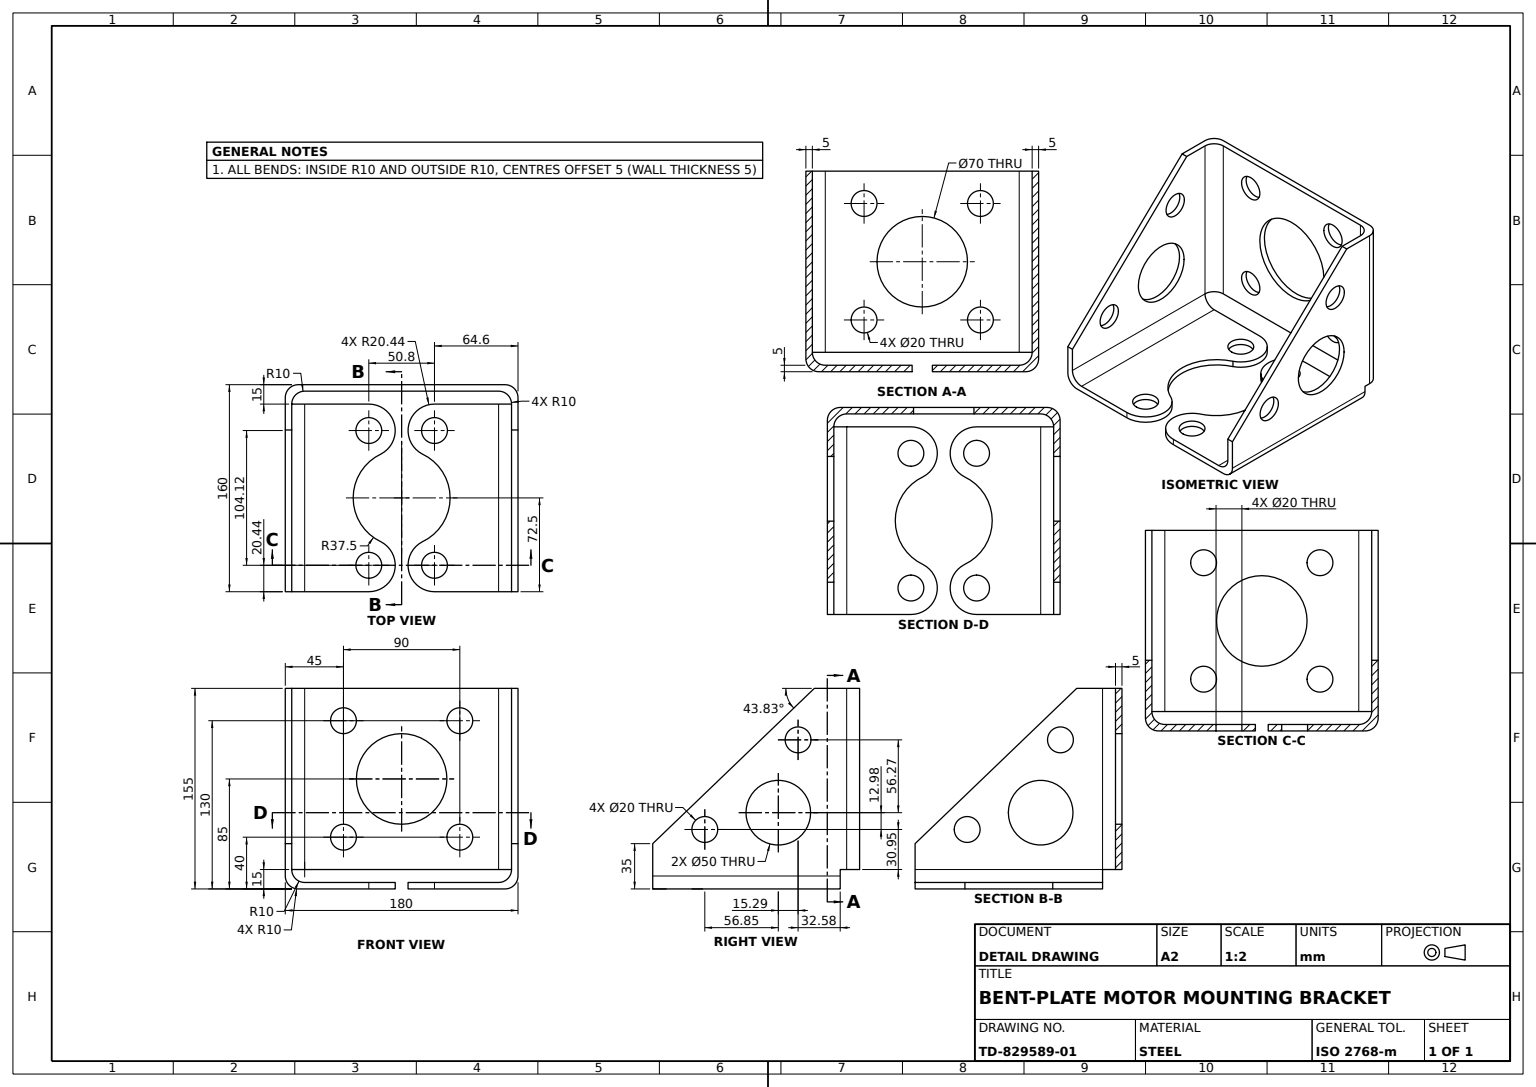
solid
v1 (75,-80,15)
v2 (85,-70,15)
e1 v1 v2 CIRCLE(AX(P(75,-70,15),D(0,0,1),D(1,0,0)),10)
v3 (75,-80,160)
e2 v3 v1 LINE
v4 (85,-70,160)
e3 v4 v3 CIRCLE(AX(P(75,-70,160),D(0,0,-1),D(-1,0,0)),10)
e4 v2 v4 LINE
face CYL(AX(P(75,-70,0),D(0,0,1),D(1,0,0)),10) rev [-e1 -e2 -e3 -e4]
v5 (-85,-26.069366,37.873409)
v6 (-90,-26.069366,37.873409)
e5 v5 v6 LINE
v7 (-85,-26.069366,87.873409)
e6 v7 v5 CIRCLE(AX(P(-85,-26.069366,62.873409),D(-1,0,0),D(0,0,1)),25)
v8 (-90,-26.069366,87.873409)
e7 v7 v8 LINE
e8 v8 v6 CIRCLE(AX(P(-90,-26.069366,62.873409),D(-1,0,0),D(0,0,1)),25)
face CYL(AX(P(-85,-26.069366,62.873409),D(-1,0,0),D(0,0,1)),25) rev [-e5 -e6 e7 e8]
v9 (-25.4,-80,129.56)
v10 (-25.4,-80,149.56)
e9 v9 v10 CIRCLE(AX(P(-25.4,-80,139.56),D(0,-1,0),D(0,0,-1)),10)
e10 v10 v9 CIRCLE(AX(P(-25.4,-80,139.56),D(0,-1,0),D(0,0,-1)),10)
v11 (-75,-80,15)
v12 (-75,-80,160)
e11 v11 v12 LINE
v13 (-25.4,-80,160)
e12 v12 v13 LINE
v14 (-15.8913,-80,121.466404)
e13 v14 v13 CIRCLE(AX(P(-25.4,-80,139.56),D(0,-1,0),D(0,0,-1)),20.44)
v15 (-15.8913,-80,53.533596)
e14 v14 v15 CIRCLE(AX(P(0,-80,87.5),D(0,-1,0),D(0,0,-1)),37.5)
v16 (-25.4,-80,15)
e15 v16 v15 CIRCLE(AX(P(-25.4,-80,35.44),D(0,-1,0),D(0,0,-1)),20.44)
e16 v11 v16 LINE
v17 (-25.4,-80,45.44)
v18 (-25.4,-80,25.44)
e17 v17 v18 CIRCLE(AX(P(-25.4,-80,35.44),D(0,-1,0),D(0,0,-1)),10)
e18 v18 v17 CIRCLE(AX(P(-25.4,-80,35.44),D(0,-1,0),D(0,0,-1)),10)
face PLANE(AX(P(0,-80,0),D(0,-1,0),D(0,0,-1))) rev [e9 e10] [e11 e12 -e13 e14 -e15 -e16] [e17 e18]
v19 (-85,-70,15)
e19 v19 v11 CIRCLE(AX(P(-75,-70,15),D(0,0,1),D(1,0,0)),10)
v20 (-85,-70,160)
e20 v20 v19 LINE
e21 v12 v20 CIRCLE(AX(P(-75,-70,160),D(0,0,-1),D(1,0,0)),10)
face CYL(AX(P(-75,-70,0),D(0,0,-1),D(-1,0,0)),10) rev [-e11 -e19 -e20 -e21]
v21 (85,-39.054338,129.718729)
v22 (90,-39.054338,129.718729)
e22 v21 v22 LINE
v23 (85,-39.054338,109.718729)
e23 v21 v23 CIRCLE(AX(P(85,-39.054338,119.718729),D(-1,0,0),D(0,0,1)),10)
v24 (90,-39.054338,109.718729)
e24 v23 v24 LINE
e25 v22 v24 CIRCLE(AX(P(90,-39.054338,119.718729),D(-1,0,0),D(0,0,1)),10)
face CYL(AX(P(85,-39.054338,119.718729),D(1,0,0),D(0,0,-1)),10) rev [-e22 e23 e24 -e25]
v25 (-85,-39.054338,109.718729)
v26 (-85,-39.054338,129.718729)
e26 v25 v26 CIRCLE(AX(P(-85,-39.054338,119.718729),D(-1,0,0),D(0,0,1)),10)
e27 v26 v25 CIRCLE(AX(P(-85,-39.054338,119.718729),D(-1,0,0),D(0,0,1)),10)
v27 (-85,70,15)
v28 (-85,70,35)
e28 v27 v28 LINE
v29 (-85,-50,160)
e29 v29 v28 LINE
e30 v20 v29 LINE
e31 v19 v27 LINE
e32 v5 v7 CIRCLE(AX(P(-85,-26.069366,62.873409),D(-1,0,0),D(0,0,1)),25)
v30 (-85,30.198845,57.579997)
v31 (-85,30.198845,37.579997)
e33 v30 v31 CIRCLE(AX(P(-85,30.198845,47.579997),D(-1,0,0),D(0,0,1)),10)
e34 v31 v30 CIRCLE(AX(P(-85,30.198845,47.579997),D(-1,0,0),D(0,0,1)),10)
face PLANE(AX(P(-85,0,0),D(-1,0,0),D(0,0,1))) rev [e26 e27] [e28 -e29 -e30 e20 e31] [e32 e6] [e33 e34]
v32 (25.4,-80,15)
e35 v32 v1 LINE
v33 (15.8913,-80,53.533596)
e36 v33 v32 CIRCLE(AX(P(25.4,-80,35.44),D(0,-1,0),D(0,0,-1)),20.44)
v34 (15.8913,-80,121.466404)
e37 v33 v34 CIRCLE(AX(P(0,-80,87.5),D(0,-1,0),D(0,0,-1)),37.5)
v35 (25.4,-80,160)
e38 v35 v34 CIRCLE(AX(P(25.4,-80,139.56),D(0,-1,0),D(0,0,-1)),20.44)
e39 v35 v3 LINE
v36 (25.4,-80,45.44)
v37 (25.4,-80,25.44)
e40 v36 v37 CIRCLE(AX(P(25.4,-80,35.44),D(0,-1,0),D(0,0,-1)),10)
e41 v37 v36 CIRCLE(AX(P(25.4,-80,35.44),D(0,-1,0),D(0,0,-1)),10)
v38 (25.4,-80,149.56)
v39 (25.4,-80,129.56)
e42 v38 v39 CIRCLE(AX(P(25.4,-80,139.56),D(0,-1,0),D(0,0,-1)),10)
e43 v39 v38 CIRCLE(AX(P(25.4,-80,139.56),D(0,-1,0),D(0,0,-1)),10)
face PLANE(AX(P(0,-80,0),D(0,-1,0),D(0,0,-1))) rev [e2 -e35 -e36 e37 -e38 e39] [e40 e41] [e42 e43]
v40 (90,-70,15)
e44 v2 v40 LINE
v41 (90,-75,15)
e45 v41 v40 LINE
v42 (80,-85,15)
e46 v41 v42 CIRCLE(AX(P(80,-75,15),D(0,0,-1),D(1,0,0)),10)
v43 (25.4,-85,15)
e47 v43 v42 LINE
e48 v32 v43 LINE
face PLANE(AX(P(85,-85,15),D(0,0,1),D(1,0,0))) rev [e35 e1 e44 -e45 e46 -e47 -e48]
v44 (-15.8913,-85,121.466404)
e49 v14 v44 LINE
v45 (-25.4,-85,160)
e50 v13 v45 LINE
e51 v44 v45 CIRCLE(AX(P(-25.4,-85,139.56),D(0,-1,0),D(0,0,-1)),20.44)
face CYL(AX(P(-25.4,-80,139.56),D(0,-1,0),D(0,0,-1)),20.44) [-e49 e13 e50 -e51]
v46 (90,-26.069366,37.873409)
v47 (90,-26.069366,87.873409)
e52 v46 v47 CIRCLE(AX(P(90,-26.069366,62.873409),D(-1,0,0),D(0,0,1)),25)
v48 (85,-26.069366,37.873409)
e53 v48 v46 LINE
v49 (85,-26.069366,87.873409)
e54 v48 v49 CIRCLE(AX(P(85,-26.069366,62.873409),D(-1,0,0),D(0,0,1)),25)
e55 v49 v47 LINE
face CYL(AX(P(85,-26.069366,62.873409),D(1,0,0),D(0,0,-1)),25) rev [-e52 -e53 e54 e55]
v50 (25.4,-85,45.44)
v51 (25.4,-85,25.44)
e56 v50 v51 CIRCLE(AX(P(25.4,-85,35.44),D(0,-1,0),D(0,0,-1)),10)
e57 v37 v51 LINE
e58 v36 v50 LINE
face CYL(AX(P(25.4,-80,35.44),D(0,-1,0),D(0,0,-1)),10) rev [e56 -e57 -e40 e58]
e59 v23 v21 CIRCLE(AX(P(85,-39.054338,119.718729),D(-1,0,0),D(0,0,1)),10)
e60 v24 v22 CIRCLE(AX(P(90,-39.054338,119.718729),D(-1,0,0),D(0,0,1)),10)
face CYL(AX(P(85,-39.054338,119.718729),D(1,0,0),D(0,0,-1)),10) rev [e59 e22 -e60 -e24]
v52 (-55,-45,5)
v53 (-35,-45,5)
e61 v52 v53 CIRCLE(AX(P(-45,-45,5),D(0,0,1),D(1,0,0)),10)
v54 (-35,-45,0)
e62 v53 v54 LINE
v55 (-55,-45,0)
e63 v55 v54 CIRCLE(AX(P(-45,-45,0),D(0,0,1),D(1,0,0)),10)
e64 v52 v55 LINE
face CYL(AX(P(-45,-45,5),D(0,0,-1),D(-1,0,0)),10) rev [e61 e62 -e63 -e64]
e65 v6 v8 CIRCLE(AX(P(-90,-26.069366,62.873409),D(-1,0,0),D(0,0,1)),25)
v56 (-90,70,35)
v57 (-90,70,10)
e66 v56 v57 LINE
v58 (-90,-70,10)
e67 v57 v58 LINE
v59 (-90,-70,15)
e68 v59 v58 LINE
v60 (-90,-75,15)
e69 v60 v59 LINE
v61 (-90,-75,160)
e70 v60 v61 LINE
v62 (-90,-50,160)
e71 v61 v62 LINE
e72 v62 v56 LINE
v63 (-90,30.198845,37.579997)
v64 (-90,30.198845,57.579997)
e73 v63 v64 CIRCLE(AX(P(-90,30.198845,47.579997),D(-1,0,0),D(0,0,1)),10)
e74 v64 v63 CIRCLE(AX(P(-90,30.198845,47.579997),D(-1,0,0),D(0,0,1)),10)
v65 (-90,-39.054338,109.718729)
v66 (-90,-39.054338,129.718729)
e75 v65 v66 CIRCLE(AX(P(-90,-39.054338,119.718729),D(-1,0,0),D(0,0,1)),10)
e76 v66 v65 CIRCLE(AX(P(-90,-39.054338,119.718729),D(-1,0,0),D(0,0,1)),10)
face PLANE(AX(P(-90,-70,5),D(1,0,0),D(0,0,-1))) rev [-e8 -e65] [e66 e67 -e68 -e69 e70 e71 e72] [-e73 -e74] [-e75 -e76]
v67 (75,-70,5)
e77 v2 v67 CIRCLE(AX(P(75,-70,15),D(0,1,0),D(0,0,1)),10)
v68 (-75,-70,5)
e78 v68 v67 LINE
e79 v68 v19 CIRCLE(AX(P(-75,-70,15),D(0,1,0),D(0,0,1)),10)
e80 v59 v19 LINE
v69 (-80,-70,0)
e81 v58 v69 CIRCLE(AX(P(-80,-70,10),D(0,-1,0),D(0,0,1)),10)
v70 (80,-70,0)
e82 v69 v70 LINE
v71 (90,-70,10)
e83 v70 v71 CIRCLE(AX(P(80,-70,10),D(0,-1,0),D(0,0,1)),10)
e84 v40 v71 LINE
face PLANE(AX(P(-90,-70,5),D(0,1,0),D(0,0,1))) rev [e77 -e78 e79 -e80 e68 e81 e82 e83 -e84 -e44]
v72 (25.4,-85,149.56)
e85 v38 v72 LINE
v73 (25.4,-85,129.56)
e86 v39 v73 LINE
e87 v73 v72 CIRCLE(AX(P(25.4,-85,139.56),D(0,-1,0),D(0,0,-1)),10)
face CYL(AX(P(25.4,-80,139.56),D(0,-1,0),D(0,0,-1)),10) rev [-e85 -e43 e86 e87]
v74 (85,30.198845,37.579997)
v75 (85,30.198845,57.579997)
e88 v74 v75 CIRCLE(AX(P(85,30.198845,47.579997),D(-1,0,0),D(0,0,1)),10)
e89 v75 v74 CIRCLE(AX(P(85,30.198845,47.579997),D(-1,0,0),D(0,0,1)),10)
v76 (85,-50,160)
e90 v4 v76 LINE
v77 (85,70,35)
e91 v76 v77 LINE
v78 (85,70,15)
e92 v78 v77 LINE
e93 v78 v2 LINE
e94 v49 v48 CIRCLE(AX(P(85,-26.069366,62.873409),D(-1,0,0),D(0,0,1)),25)
face PLANE(AX(P(85,0,0),D(-1,0,0),D(0,0,1))) [-e88 -e89] [e90 e91 -e92 e93 e4] [-e23 -e59] [-e94 -e54]
e95 v30 v64 LINE
e96 v31 v63 LINE
face CYL(AX(P(-85,30.198845,47.579997),D(-1,0,0),D(0,0,1)),10) rev [-e95 -e34 e96 e73]
v79 (-25.4,-85,149.56)
e97 v10 v79 LINE
v80 (-25.4,-85,129.56)
e98 v9 v80 LINE
e99 v80 v79 CIRCLE(AX(P(-25.4,-85,139.56),D(0,-1,0),D(0,0,-1)),10)
face CYL(AX(P(-25.4,-80,139.56),D(0,-1,0),D(0,0,-1)),10) rev [-e97 -e9 e98 e99]
e100 v53 v52 CIRCLE(AX(P(-45,-45,5),D(0,0,1),D(1,0,0)),10)
e101 v54 v55 CIRCLE(AX(P(-45,-45,0),D(0,0,1),D(1,0,0)),10)
face CYL(AX(P(-45,-45,5),D(0,0,-1),D(-1,0,0)),10) rev [-e62 e100 e64 -e101]
v81 (55,-45,0)
v82 (35,-45,0)
e102 v81 v82 CIRCLE(AX(P(45,-45,0),D(0,0,1),D(1,0,0)),10)
v83 (55,-45,5)
e103 v83 v81 LINE
v84 (35,-45,5)
e104 v83 v84 CIRCLE(AX(P(45,-45,5),D(0,0,1),D(1,0,0)),10)
e105 v84 v82 LINE
face CYL(AX(P(45,-45,5),D(0,0,-1),D(-1,0,0)),10) rev [-e102 -e103 e104 e105]
v85 (-80,-85,160)
e106 v61 v85 CIRCLE(AX(P(-80,-75,160),D(0,0,1),D(1,0,0)),10)
e107 v45 v85 LINE
e108 v29 v62 LINE
face PLANE(AX(P(-85,0,160),D(0,0,1),D(1,0,0))) [e106 -e107 -e50 -e12 e21 e30 e108 -e71]
v86 (-55,45,0)
v87 (-35,45,0)
e109 v86 v87 CIRCLE(AX(P(-45,45,0),D(0,0,1),D(1,0,0)),10)
e110 v87 v86 CIRCLE(AX(P(-45,45,0),D(0,0,1),D(1,0,0)),10)
v88 (80,70,0)
v89 (-80,70,0)
e111 v88 v89 LINE
e112 v88 v70 LINE
e113 v69 v89 LINE
e114 v82 v81 CIRCLE(AX(P(45,-45,0),D(0,0,1),D(1,0,0)),10)
v90 (35,0,0)
v91 (-35,0,0)
e115 v90 v91 CIRCLE(AX(P(0,0,0),D(0,0,1),D(1,0,0)),35)
e116 v91 v90 CIRCLE(AX(P(0,0,0),D(0,0,1),D(1,0,0)),35)
v92 (35,45,0)
v93 (55,45,0)
e117 v92 v93 CIRCLE(AX(P(45,45,0),D(0,0,1),D(1,0,0)),10)
e118 v93 v92 CIRCLE(AX(P(45,45,0),D(0,0,1),D(1,0,0)),10)
face PLANE(AX(P(0,0,0),D(0,0,-1),D(-1,0,0))) [e109 e110] [e101 e63] [-e111 e112 -e82 e113] [e114 e102] [e115 e116] [e117 e118]
v94 (-25.4,-85,45.44)
v95 (-25.4,-85,25.44)
e119 v94 v95 CIRCLE(AX(P(-25.4,-85,35.44),D(0,-1,0),D(0,0,-1)),10)
e120 v18 v95 LINE
e121 v17 v94 LINE
face CYL(AX(P(-25.4,-80,35.44),D(0,-1,0),D(0,0,-1)),10) rev [e119 -e120 -e17 e121]
e122 v72 v73 CIRCLE(AX(P(25.4,-85,139.56),D(0,-1,0),D(0,0,-1)),10)
face CYL(AX(P(25.4,-80,139.56),D(0,-1,0),D(0,0,-1)),10) rev [e122 -e86 -e42 e85]
v96 (90,-75,160)
e123 v96 v41 LINE
v97 (80,-85,160)
e124 v97 v96 CIRCLE(AX(P(80,-75,160),D(0,0,1),D(-1,0,0)),10)
e125 v42 v97 LINE
face CYL(AX(P(80,-75,0),D(0,0,-1),D(-1,0,0)),10) [-e123 -e124 -e125 -e46]
v98 (90,30.198845,57.579997)
e126 v75 v98 LINE
v99 (90,30.198845,37.579997)
e127 v99 v98 CIRCLE(AX(P(90,30.198845,47.579997),D(-1,0,0),D(0,0,1)),10)
e128 v74 v99 LINE
face CYL(AX(P(85,30.198845,47.579997),D(1,0,0),D(0,0,-1)),10) rev [e126 -e127 -e128 e88]
v100 (35,45,5)
e129 v100 v92 LINE
v101 (55,45,5)
e130 v100 v101 CIRCLE(AX(P(45,45,5),D(0,0,1),D(1,0,0)),10)
e131 v101 v93 LINE
face CYL(AX(P(45,45,5),D(0,0,-1),D(-1,0,0)),10) rev [-e129 e130 e131 -e117]
e132 v95 v94 CIRCLE(AX(P(-25.4,-85,35.44),D(0,-1,0),D(0,0,-1)),10)
face CYL(AX(P(-25.4,-80,35.44),D(0,-1,0),D(0,0,-1)),10) rev [e120 e132 -e121 -e18]
e133 v89 v57 CIRCLE(AX(P(-80,70,10),D(0,1,0),D(0,0,-1)),10)
face CYL(AX(P(-80,-70,10),D(0,1,0),D(0,0,1)),10) [-e81 -e67 -e133 -e113]
v102 (-15.8913,-85,53.533596)
e134 v44 v102 CIRCLE(AX(P(0,-85,87.5),D(0,-1,0),D(0,0,-1)),37.5)
v103 (-80,-85,15)
e135 v85 v103 LINE
v104 (-25.4,-85,15)
e136 v103 v104 LINE
e137 v104 v102 CIRCLE(AX(P(-25.4,-85,35.44),D(0,-1,0),D(0,0,-1)),20.44)
e138 v79 v80 CIRCLE(AX(P(-25.4,-85,139.56),D(0,-1,0),D(0,0,-1)),10)
face PLANE(AX(P(0,-85,0),D(0,-1,0),D(0,0,-1))) [-e132 -e119] [-e134 e51 e107 e135 e136 e137] [-e99 -e138]
e139 v26 v66 LINE
e140 v25 v65 LINE
face CYL(AX(P(-85,-39.054338,119.718729),D(-1,0,0),D(0,0,1)),10) rev [e75 -e139 -e26 e140]
e141 v101 v100 CIRCLE(AX(P(45,45,5),D(0,0,1),D(1,0,0)),10)
face CYL(AX(P(45,45,5),D(0,0,-1),D(-1,0,0)),10) rev [e141 e129 -e118 -e131]
v105 (-35,45,5)
v106 (-55,45,5)
e142 v105 v106 CIRCLE(AX(P(-45,45,5),D(0,0,1),D(1,0,0)),10)
e143 v106 v86 LINE
e144 v105 v87 LINE
face CYL(AX(P(-45,45,5),D(0,0,-1),D(-1,0,0)),10) rev [e142 e143 -e110 -e144]
e145 v84 v83 CIRCLE(AX(P(45,-45,5),D(0,0,1),D(1,0,0)),10)
face CYL(AX(P(45,-45,5),D(0,0,-1),D(-1,0,0)),10) rev [-e105 e145 e103 -e114]
e146 v103 v60 CIRCLE(AX(P(-80,-75,15),D(0,0,-1),D(1,0,0)),10)
face CYL(AX(P(-80,-75,0),D(0,0,1),D(1,0,0)),10) [-e70 -e146 -e135 -e106]
v107 (25.4,-85,160)
v108 (15.8913,-85,121.466404)
e147 v107 v108 CIRCLE(AX(P(25.4,-85,139.56),D(0,-1,0),D(0,0,-1)),20.44)
e148 v35 v107 LINE
e149 v34 v108 LINE
face CYL(AX(P(25.4,-80,139.56),D(0,-1,0),D(0,0,-1)),20.44) [-e147 -e148 e38 e149]
face CYL(AX(P(-25.4,-80,139.56),D(0,-1,0),D(0,0,-1)),10) rev [-e98 -e10 e97 e138]
v109 (90,70,35)
e150 v77 v109 LINE
v110 (90,-50,160)
e151 v76 v110 LINE
e152 v110 v109 LINE
face PLANE(AX(P(85,17.843464,89.329725),D(0,-0.721387321,-0.692531828),D(0,0.692531828,-0.721387321))) rev [-e150 -e91 e151 e152]
v111 (15.8913,-85,53.533596)
e153 v33 v111 LINE
e154 v111 v43 CIRCLE(AX(P(25.4,-85,35.44),D(0,-1,0),D(0,0,-1)),20.44)
face CYL(AX(P(25.4,-80,35.44),D(0,-1,0),D(0,0,-1)),20.44) [-e153 e36 e48 -e154]
v112 (-75,70,5)
e155 v27 v112 CIRCLE(AX(P(-75,70,15),D(0,-1,0),D(0,0,-1)),10)
e156 v112 v68 LINE
face CYL(AX(P(-75,0,15),D(0,-1,0),D(0,0,-1)),10) rev [-e155 -e31 -e79 -e156]
e157 v111 v108 CIRCLE(AX(P(0,-85,87.5),D(0,-1,0),D(0,0,-1)),37.5)
face CYL(AX(P(0,-80,87.5),D(0,-1,0),D(0,0,-1)),37.5) rev [-e37 e153 e157 -e149]
e158 v51 v50 CIRCLE(AX(P(25.4,-85,35.44),D(0,-1,0),D(0,0,-1)),10)
e159 v97 v107 LINE
face PLANE(AX(P(0,-85,0),D(0,-1,0),D(0,0,-1))) [-e56 -e158] [-e87 -e122] [e125 e159 e147 -e157 e154 e47]
e160 v16 v104 LINE
e161 v15 v102 LINE
face CYL(AX(P(-25.4,-80,35.44),D(0,-1,0),D(0,0,-1)),20.44) [-e137 -e160 e15 e161]
e162 v47 v46 CIRCLE(AX(P(90,-26.069366,62.873409),D(-1,0,0),D(0,0,1)),25)
face CYL(AX(P(85,-26.069366,62.873409),D(1,0,0),D(0,0,-1)),25) rev [-e162 -e55 e94 e53]
v113 (90,70,10)
e163 v71 v113 LINE
e164 v113 v88 CIRCLE(AX(P(80,70,10),D(0,1,0),D(0,0,-1)),10)
face CYL(AX(P(80,-70,10),D(0,-1,0),D(0,0,-1)),10) [-e163 -e83 -e112 -e164]
face PLANE(AX(P(-90,-85,15),D(0,0,1),D(1,0,0))) rev [e16 e160 -e136 e146 e69 e80 e19]
face CYL(AX(P(-85,-39.054338,119.718729),D(-1,0,0),D(0,0,1)),10) rev [-e27 e139 e76 -e140]
e165 v98 v99 CIRCLE(AX(P(90,30.198845,47.579997),D(-1,0,0),D(0,0,1)),10)
face CYL(AX(P(85,30.198845,47.579997),D(1,0,0),D(0,0,-1)),10) rev [-e165 -e126 e89 e128]
v114 (75,70,5)
e166 v114 v78 CIRCLE(AX(P(75,70,15),D(0,-1,0),D(0,0,-1)),10)
e167 v67 v114 LINE
face CYL(AX(P(75,0,15),D(0,1,0),D(0,0,1)),10) rev [-e166 -e167 -e77 -e93]
e168 v96 v110 LINE
face PLANE(AX(P(85,-70,160),D(0,0,-1),D(-1,0,0))) rev [-e39 e148 -e159 e124 e168 -e151 -e90 e3]
e169 v106 v105 CIRCLE(AX(P(-45,45,5),D(0,0,1),D(1,0,0)),10)
e170 v114 v112 LINE
v115 (35,0,5)
v116 (-35,0,5)
e171 v115 v116 CIRCLE(AX(P(0,0,5),D(0,0,1),D(1,0,0)),35)
e172 v116 v115 CIRCLE(AX(P(0,0,5),D(0,0,1),D(1,0,0)),35)
face PLANE(AX(P(0,0,5),D(0,0,-1),D(-1,0,0))) rev [-e104 -e145] [-e169 -e142] [e167 e170 e156 e78] [-e171 -e172] [-e100 -e61] [-e130 -e141]
e173 v109 v113 LINE
face PLANE(AX(P(90,-70,5),D(-1,0,0),D(0,0,1))) rev [-e152 -e168 e123 e45 e84 e163 -e173] [e52 e162] [e165 e127] [e25 e60]
face CYL(AX(P(-85,-26.069366,62.873409),D(-1,0,0),D(0,0,1)),25) rev [e5 e65 -e7 -e32]
e174 v116 v91 LINE
e175 v115 v90 LINE
face CYL(AX(P(0,0,5),D(0,0,-1),D(-1,0,0)),35) rev [e171 e174 -e115 -e175]
e176 v28 v56 LINE
face PLANE(AX(P(-85,53.913405,51.756869),D(0,0.721387321,0.692531828),D(0,-0.692531828,0.721387321))) [e176 -e72 -e108 e29]
face PLANE(AX(P(-90,70,5),D(0,-1,0),D(0,0,-1))) rev [e166 e92 e150 e173 e164 e111 e133 -e66 -e176 -e28 e155 -e170]
face CYL(AX(P(0,-80,87.5),D(0,-1,0),D(0,0,-1)),37.5) rev [e49 e134 -e161 -e14]
face CYL(AX(P(25.4,-80,35.44),D(0,-1,0),D(0,0,-1)),10) rev [e158 -e58 -e41 e57]
face CYL(AX(P(-85,30.198845,47.579997),D(-1,0,0),D(0,0,1)),10) rev [-e33 e95 e74 -e96]
face CYL(AX(P(-45,45,5),D(0,0,-1),D(-1,0,0)),10) rev [e144 -e109 -e143 e169]
face CYL(AX(P(0,0,5),D(0,0,-1),D(-1,0,0)),35) rev [-e116 -e174 e172 e175]
